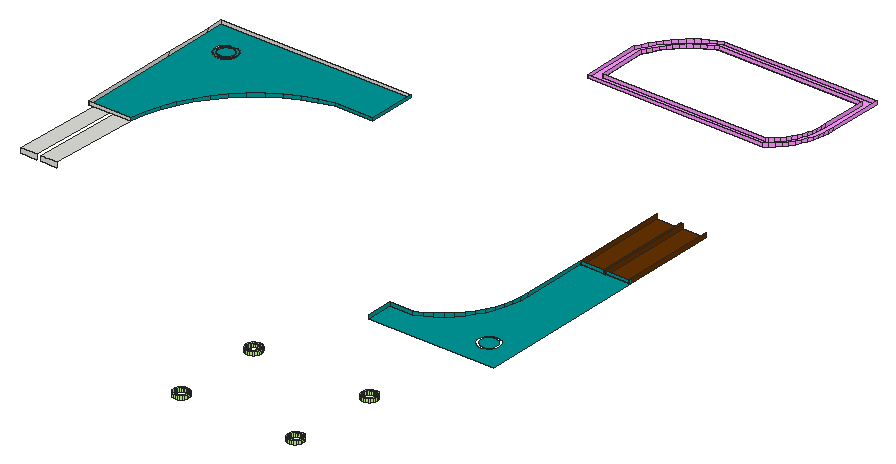
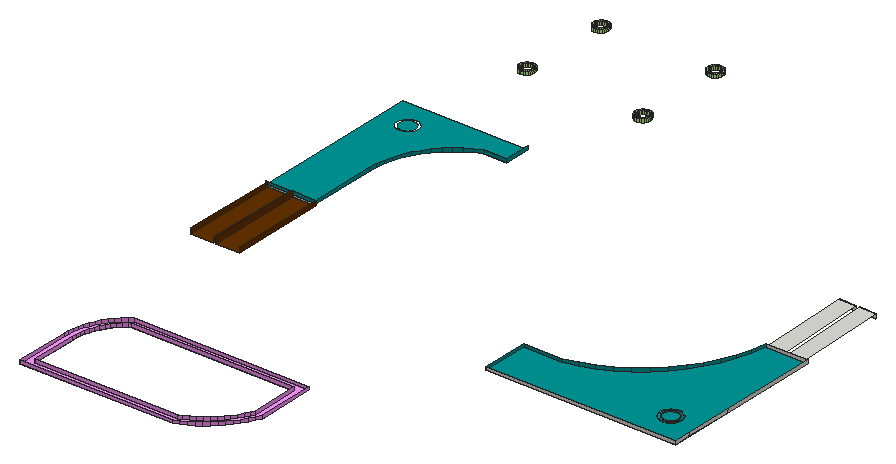
# SketchUp Ruby script. Lengths in inches.
U = 1.inch
M = Sketchup.active_model
def pt(a) = Geom::Point3d.new(a.map { |v| v * U })
def face(e, loops, mat)
  f = e.add_face(loops[0].map { |a| pt(a) })
  loops[1..].each { |l| e.add_face(l.map { |a| pt(a) }).erase! }
  f.material = f.back_material = mat if mat
  f
end
# faces: each face lists its corners as indices into pts; further lists are holes
def faces(e, pts, list, mat = nil) = list.each { |f| face(e, (f[0].is_a?(Array) ? f : [f]).map { |l| l.map { |i| pts[i] } }, mat) }
# xy, xz, yz: faces in a plane at the given z, y or x. An outline is a flat list of corners, or four numbers for a rectangle; further outlines are holes
def ring(l) = l.size == 4 ? [[l[0], l[1]], [l[2], l[1]], [l[2], l[3]], [l[0], l[3]]] : l.each_slice(2).to_a
def flat(e, list, mat, &to3) = list.each { |f| face(e, (f[0].is_a?(Array) ? f : [f]).map { |l| ring(l).map { |u, v| to3.(u, v) } }, mat) }
def xy(e, z, list, mat = nil) = flat(e, list, mat) { |x, y| [x, y, z] }
def xz(e, y, list, mat = nil) = flat(e, list, mat) { |x, z| [x, y, z] }
def yz(e, x, list, mat = nil) = flat(e, list, mat) { |y, z| [x, y, z] }
def lines(e, pts, list) = list.each { |a, b| e.add_line(pt(pts[a]), pt(pts[b])) }
# prism: a flat outline (further loops are holes) pulled along v
def prism(e, loops, v, mat = nil)
  f = face(e, loops, mat); d = Geom::Vector3d.new(v.map { |x| x * U })
  f.pushpull(f.normal.samedirection?(d) ? d.length : -d.length)
end
def box(e, o, s, mat = nil) = prism(e, [[o, [o[0] + s[0], o[1], o[2]], [o[0] + s[0], o[1] + s[1], o[2]], [o[0], o[1] + s[1], o[2]]]], [0, 0, s[2]], mat)
def at(x, y, z, deg = 0) = Geom::Transformation.translation(pt([x, y, z])) * Geom::Transformation.rotation(ORIGIN, Z_AXIS, deg.degrees)
def axes(o, x, y, z) = Geom::Transformation.new([*x, 0, *y, 0, *z, 0, *pt(o).to_a, 1])
def part(name) = M.definitions.add(name)
# library, detail: a bought-in or finely detailed component or shape, given as its bounding box
def library(name, o, s) = part(name).tap { |d| box(d.entities, o, s) }
def detail(e, o, s) = box(e.add_group.entities, o, s)
def put(e, d, t, mat = nil) = e.add_instance(d, t).tap { |i| i.material = mat if mat }
def group(e, t, mat = nil) = e.add_group.tap { |g| g.transformation = t; g.material = mat if mat }.entities
root = M.entities
M.materials.add("[Color C08]").color = [102, 51, 0]
M.materials.add("[Color F02]").color = [204, 255, 153]
M.materials.add("[Color H07]").color = [0, 153, 153]
M.materials.add("[Color K02]").color = [255, 153, 255]
M.materials.add("[Color M00]").color = [255, 255, 255]
M.materials.add("[Marble Carrara Gold Floor Tile]").color = [225, 223, 217]
xy(root,116.1875,[[418.74,309.14,433.17,368.58],[434.49,309.14,448.92,368.58]],"[Color C08]")
xy(root,116.1875,[[[153.48,358.9,151.72,358.91,150.02,359.37,148.49,360.26,147.25,361.51,146.375,363.04,145.93,364.74,145.93,366.51,146.4,368.21,147.28,369.73,148.53,370.97,150.0625,371.85,151.77,372.29,153.53,372.29,155.23,371.83,156.75,370.9375,157.99,369.6875,158.87,368.16,159.32,366.45,159.3125,364.69,158.85,362.99,157.96,361.47,156.71,360.23,155.18,359.35],[152.62,360.6,153.92,360.77,155.12,361.27,156.16,362.0625,156.95,363.1,157.45,364.31,157.62,365.6,157.45,366.89,156.95,368.1,156.16,369.13,155.12,369.93,153.92,370.43,152.62,370.6,151.33,370.43,150.12,369.93,149.09,369.13,148.29,368.1,147.79,366.89,147.62,365.6,147.79,364.31,148.29,363.1,149.09,362.0625,150.12,361.27,151.33,360.77]]],"[Color M00]")
xy(root,117.1875,[[[348.25,81.79,347.02,81.91,345.85,82.34,344.84,83.06,344.05,84.01,343.53,85.14,343.33,86.36,343.44,87.6,343.875,88.76,344.59,89.77,345.55,90.5625,346.68,91.08,347.9,91.29,349.13,91.17,350.29,90.74,351.31,90.02,352.1,89.07,352.61,87.9375,352.82,86.72,352.7,85.48,352.27,84.32,351.55,83.31,350.6,82.52,349.47,82],[348.07,83.14,348.95,83.26,349.77,83.6,350.48,84.14,351.02,84.84,351.36,85.66,351.47,86.54,351.36,87.42,351.02,88.24,350.48,88.94,349.77,89.48,348.95,89.82,348.07,89.9375,347.19,89.82,346.375,89.48,345.67,88.94,345.13,88.24,344.79,87.42,344.68,86.54,344.79,85.66,345.13,84.84,345.67,84.14,346.375,83.6,347.19,83.26]],[[419.3125,81.79,418.08,81.91,416.92,82.34,415.9,83.06,415.11,84.01,414.6,85.14,414.39,86.36,414.51,87.6,414.9375,88.76,415.66,89.77,416.61,90.5625,417.74,91.08,418.96,91.29,420.2,91.17,421.36,90.74,422.37,90.02,423.16,89.07,423.68,87.9375,423.88,86.72,423.77,85.48,423.33,84.32,422.62,83.31,421.66,82.52,420.53,82],[419.14,83.14,420.02,83.26,420.84,83.6,421.54,84.14,422.08,84.84,422.42,85.66,422.53,86.54,422.42,87.42,422.08,88.24,421.54,88.94,420.84,89.48,420.02,89.82,419.14,89.9375,418.26,89.82,417.4375,89.48,416.73,88.94,416.19,88.24,415.85,87.42,415.74,86.54,415.85,85.66,416.19,84.84,416.73,84.14,417.4375,83.6,418.26,83.26]],[[421.43,136.83,420.2,136.95,419.04,137.38,418.03,138.1,417.24,139.05,416.72,140.18,416.51,141.4,416.63,142.64,417.06,143.8,417.78,144.81,418.73,145.6,419.86,146.12,421.08,146.32,422.32,146.21,423.48,145.78,424.49,145.06,425.28,144.1,425.8,142.97,426.01,141.75,425.89,140.52,425.46,139.36,424.74,138.34,423.78,137.55,422.66,137.04],[421.26,138.18,422.14,138.29,422.96,138.63,423.66,139.17,424.2,139.88,424.54,140.7,424.66,141.58,424.54,142.46,424.2,143.28,423.66,143.98,422.96,144.52,422.14,144.86,421.26,144.97,420.38,144.86,419.56,144.52,418.86,143.98,418.32,143.28,417.98,142.46,417.86,141.58,417.98,140.7,418.32,139.88,418.86,139.17,419.56,138.63,420.38,138.29]],[[348.25,138.17,347.02,138.28,345.85,138.72,344.84,139.43,344.05,140.39,343.53,141.52,343.33,142.74,343.44,143.97,343.875,145.14,344.59,146.15,345.55,146.9375,346.68,147.45,347.9,147.66,349.13,147.55,350.29,147.11,351.31,146.4,352.1,145.44,352.61,144.3125,352.82,143.09,352.7,141.86,352.27,140.69,351.55,139.68,350.6,138.89,349.47,138.375],[348.07,139.52,348.95,139.63,349.77,139.97,350.48,140.51,351.02,141.22,351.36,142.04,351.47,142.91,351.36,143.79,351.02,144.61,350.48,145.32,349.77,145.86,348.95,146.2,348.07,146.3125,347.19,146.2,346.375,145.86,345.67,145.32,345.13,144.61,344.79,143.79,344.68,142.91,344.79,142.04,345.13,141.22,345.67,140.51,346.375,139.97,347.19,139.63]]],"[Color F02]")
xy(root,117.1875,[[[371.8,202.59,371.8,218.96,386.375,218.96,391.03,221.23,395.45,223.95,399.59,227.09,403.4,230.61,406.85,234.48,409.91,238.67,412.55,243.13,414.74,247.83,416.47,252.72,417.72,257.76,418.47,262.89,418.72,268.07,418.72,309.14,449.85,309.14,449.85,202.59],[433.35,213.79,435.05,214.24,436.58,215.12,437.83,216.36,438.72,217.88,439.18,219.58,439.19,221.35,438.74,223.05,437.87,224.58,436.625,225.83,435.1,226.72,433.4,227.18,431.64,227.19,429.94,226.74,428.41,225.86,427.16,224.62,426.27,223.1,425.81,221.4,425.8,219.63,426.25,217.93,427.125,216.4,428.36,215.15,429.89,214.26,431.59,213.8]],[432.49,215.49,431.2,215.66,429.99,216.16,428.96,216.95,428.16,217.99,427.66,219.2,427.49,220.49,427.66,221.78,428.16,222.99,428.96,224.03,429.99,224.82,431.2,225.32,432.49,225.49,433.79,225.32,434.99,224.82,436.03,224.03,436.82,222.99,437.32,221.78,437.49,220.49,437.32,219.2,436.82,217.99,436.03,216.95,434.99,216.16,433.79,215.66],[[133.15,283.41,133.15,386.28,251.25,386.28,251.25,356.85,227.25,356.85,218.64,354.61,210.31,351.49,202.34,347.53,194.83,342.76,187.85,337.25,181.48,331.04,175.78,324.21,170.82,316.82,166.65,308.96,163.32,300.72,160.85,292.17,159.28,283.41],[153.48,358.9,155.18,359.35,156.71,360.23,157.96,361.47,158.85,362.99,159.3125,364.69,159.32,366.45,158.87,368.16,157.99,369.6875,156.75,370.9375,155.23,371.83,153.53,372.29,151.77,372.29,150.0625,371.85,148.53,370.97,147.28,369.73,146.4,368.21,145.93,366.51,145.93,364.74,146.375,363.04,147.25,361.51,148.49,360.26,150.02,359.37,151.72,358.91]],[[153.48,358.9,155.18,359.35,156.71,360.23,157.96,361.47,158.85,362.99,159.3125,364.69,159.32,366.45,158.87,368.16,157.99,369.6875,156.75,370.9375,155.23,371.83,153.53,372.29,151.77,372.29,150.0625,371.85,148.53,370.97,147.28,369.73,146.4,368.21,145.93,366.51,145.93,364.74,146.375,363.04,147.25,361.51,148.49,360.26,150.02,359.37,151.72,358.91],[152.62,360.6,151.33,360.77,150.12,361.27,149.09,362.0625,148.29,363.1,147.79,364.31,147.62,365.6,147.79,366.89,148.29,368.1,149.09,369.13,150.12,369.93,151.33,370.43,152.62,370.6,153.92,370.43,155.12,369.93,156.16,369.13,156.95,368.1,157.45,366.89,157.62,365.6,157.45,364.31,156.95,363.1,156.16,362.0625,155.12,361.27,153.92,360.77]],[152.62,360.6,151.33,360.77,150.12,361.27,149.09,362.0625,148.29,363.1,147.79,364.31,147.62,365.6,147.79,366.89,148.29,368.1,149.09,369.13,150.12,369.93,151.33,370.43,152.62,370.6,153.92,370.43,155.12,369.93,156.16,369.13,156.95,368.1,157.45,366.89,157.62,365.6,157.45,364.31,156.95,363.1,156.16,362.0625,155.12,361.27,153.92,360.77]],"[Color H07]")
xy(root,117.1875,[[[306.15,455.42,306.15,491.45,307.65,494.89,309.39,498.21,311.35,501.41,313.52,504.47,315.89,507.38,318.45,510.12,321.1875,512.68,324.1,515.05,327.16,517.22,330.36,519.18,333.68,520.92,337.12,522.42,432.08,522.42,432.08,488.92,431.95,485.67,431.57,482.43,430.93,479.23,430.04,476.1,428.9,473.04,427.52,470.09,425.92,467.25,424.1,464.55,422.07,462,419.84,459.62,417.43,457.42,414.86,455.42],[311.23,460.51,413.12,460.51,414.15,461.3125,416.27,463.24,418.22,465.33,420,467.5625,421.59,469.93,423,472.42,424.2,475.01,425.2,477.68,425.98,480.43,426.54,483.23,426.88,486.07,427,489.02,427,517.34,338.18,517.34,335.88,516.33,332.86,514.75,329.96,512.97,327.18,511,324.53,508.85,322.05,506.52,319.72,504.03,317.57,501.39,315.59,498.61,313.82,495.71,312.24,492.6875,311.23,490.39]]],"[Color K02]")
xz(root,218.96,[[371.8,117.1875,386.375,119.1875]],"[Color H07]")
xz(root,283.41,[[133.15,117.1875,159.28,119.1875]],"[Marble Carrara Gold Floor Tile]")
xz(root,309.14,[[418.72,117.1875,418.74,119.1875],[418.74,117.1875,433.17,119.1875],[433.17,117.1875,434.49,119.1875],[434.49,117.1875,448.92,119.1875],[448.92,117.1875,449.85,119.1875]],"[Color H07]")
xz(root,309.14,[[418.74,116.1875,433.17,117.1875],[434.49,116.1875,448.92,117.1875]],"[Marble Carrara Gold Floor Tile]")
xz(root,356.85,[[227.25,117.1875,251.25,119.1875]],"[Color H07]")
xz(root,372.29,[[151.77,116.1875,153.53,117.1875]],"[Color M00]")
xz(root,386.28,[[133.15,117.1875,251.25,119.1875]],"[Marble Carrara Gold Floor Tile]")
xz(root,455.42,[[306.15,117.1875,414.86,119.1875]],"[Color K02]")
xz(root,460.51,[[311.23,117.1875,413.12,119.1875]],"[Color K02]")
xz(root,517.34,[[338.18,117.1875,427,119.1875]],"[Color K02]")
xz(root,522.42,[[337.12,117.1875,432.08,119.1875]],"[Color K02]")
yz(root,133.15,[[283.41,117.1875,345.53,119.1875],[345.53,117.1875,375.53,119.1875],[375.53,117.1875,386.28,119.1875]],"[Marble Carrara Gold Floor Tile]")
yz(root,145.93,[[364.74,116.1875,366.51,117.1875]],"[Color M00]")
yz(root,251.25,[[356.85,117.1875,386.28,119.1875]],"[Color H07]")
yz(root,306.15,[[455.42,117.1875,491.45,119.1875]],"[Color K02]")
yz(root,311.23,[[460.51,117.1875,490.39,119.1875]],"[Color K02]")
yz(root,371.8,[[202.59,117.1875,218.96,119.1875]],"[Color H07]")
yz(root,418.72,[[268.07,117.1875,309.14,119.1875]],"[Color H07]")
yz(root,418.74,[[309.14,116.1875,368.58,119.1875]],"[Color C08]")
yz(root,427,[[489.02,117.1875,517.34,119.1875]],"[Color K02]")
yz(root,432.08,[[488.92,117.1875,522.42,119.1875]],"[Color K02]")
yz(root,433.17,[[309.14,116.1875,368.58,119.1875]],"[Color C08]")
yz(root,434.49,[[309.14,116.1875,368.58,119.1875]],"[Color C08]")
yz(root,448.92,[[309.14,116.1875,368.58,119.1875]],"[Color C08]")
p = [[146.22,226.59,119.1875],[135.92,226.59,119.1875],[135.92,226.48,116.1875],[146.22,226.48,116.1875],[158.84,226.59,119.1875],[148.55,226.59,119.1875],
  [148.55,226.48,116.1875],[158.84,226.48,116.1875],[151.72,358.91,117.1875],[150.02,359.37,117.1875],[150.02,359.37,116.1875],[151.72,358.91,116.1875],
  [153.48,358.9,117.1875],[153.48,358.9,116.1875],[155.18,359.35,117.1875],[155.18,359.35,116.1875],[148.49,360.26,117.1875],[148.49,360.26,116.1875],
  [156.71,360.23,117.1875],[156.71,360.23,116.1875],[157.96,361.47,117.1875],[157.96,361.47,116.1875],[147.25,361.51,117.1875],[147.25,361.51,116.1875],
  [151.33,360.77,117.1875],[152.62,360.6,117.1875],[152.62,360.6,116.1875],[151.33,360.77,116.1875],[153.92,360.77,117.1875],[153.92,360.77,116.1875],
  [150.12,361.27,117.1875],[150.12,361.27,116.1875],[155.12,361.27,117.1875],[155.12,361.27,116.1875],[149.09,362.0625,117.1875],[149.09,362.0625,116.1875],
  [156.16,362.0625,117.1875],[156.16,362.0625,116.1875],[146.375,363.04,117.1875],[146.375,363.04,116.1875],[158.85,362.99,117.1875],[158.85,362.99,116.1875],
  [148.29,363.1,117.1875],[148.29,363.1,116.1875],[156.95,363.1,117.1875],[156.95,363.1,116.1875],[145.93,364.74,117.1875],[145.93,364.74,116.1875],
  [159.3125,364.69,117.1875],[159.3125,364.69,116.1875],[147.79,364.31,117.1875],[147.79,364.31,116.1875],[157.45,364.31,117.1875],[157.45,364.31,116.1875],
  [147.62,365.6,117.1875],[147.62,365.6,116.1875],[157.62,365.6,117.1875],[157.62,365.6,116.1875],[159.32,366.45,117.1875],[159.32,366.45,116.1875],
  [147.79,366.89,117.1875],[147.79,366.89,116.1875],[157.45,366.89,117.1875],[157.45,366.89,116.1875],[145.93,366.51,117.1875],[146.4,368.21,117.1875],
  [146.4,368.21,116.1875],[145.93,366.51,116.1875],[158.87,368.16,117.1875],[158.87,368.16,116.1875],[148.29,368.1,117.1875],[148.29,368.1,116.1875],
  [156.95,368.1,117.1875],[156.95,368.1,116.1875],[149.09,369.13,117.1875],[149.09,369.13,116.1875],[156.16,369.13,117.1875],[156.16,369.13,116.1875],
  [147.28,369.73,117.1875],[147.28,369.73,116.1875],[157.99,369.6875,117.1875],[157.99,369.6875,116.1875],[150.12,369.93,117.1875],[150.12,369.93,116.1875],
  [155.12,369.93,117.1875],[155.12,369.93,116.1875],[148.53,370.97,117.1875],[148.53,370.97,116.1875],[156.75,370.9375,117.1875],[156.75,370.9375,116.1875],
  [151.33,370.43,117.1875],[151.33,370.43,116.1875],[153.92,370.43,117.1875],[153.92,370.43,116.1875],[152.62,370.6,117.1875],[152.62,370.6,116.1875],
  [155.23,371.83,117.1875],[155.23,371.83,116.1875],[150.0625,371.85,117.1875],[150.0625,371.85,116.1875],[151.77,372.29,117.1875],[151.77,372.29,116.1875],
  [153.53,372.29,117.1875],[153.53,372.29,116.1875],[135.92,287.31,116.99],[146.22,287.31,116.99],[148.55,286.68,117.02],[158.84,286.68,117.02],
  [348.25,81.79,119.1875],[347.02,81.91,119.1875],[347.02,81.91,117.1875],[348.25,81.79,117.1875],[349.47,82,119.1875],[349.47,82,117.1875],
  [419.3125,81.79,119.1875],[418.08,81.91,119.1875],[418.08,81.91,117.1875],[419.3125,81.79,117.1875],[420.53,82,119.1875],[420.53,82,117.1875],
  [345.85,82.34,119.1875],[345.85,82.34,117.1875],[416.92,82.34,119.1875],[416.92,82.34,117.1875],[350.6,82.52,119.1875],[350.6,82.52,117.1875],
  [421.66,82.52,119.1875],[421.66,82.52,117.1875],[344.84,83.06,119.1875],[344.84,83.06,117.1875],[415.9,83.06,119.1875],[415.9,83.06,117.1875],
  [351.55,83.31,119.1875],[351.55,83.31,117.1875],[422.62,83.31,119.1875],[422.62,83.31,117.1875],[344.05,84.01,119.1875],[344.05,84.01,117.1875],
  [347.19,83.26,119.1875],[348.07,83.14,119.1875],[348.07,83.14,117.1875],[347.19,83.26,117.1875],[348.95,83.26,119.1875],[348.95,83.26,117.1875],
  [415.11,84.01,119.1875],[415.11,84.01,117.1875],[418.26,83.26,119.1875],[419.14,83.14,119.1875],[419.14,83.14,117.1875],[418.26,83.26,117.1875],
  [420.02,83.26,119.1875],[420.02,83.26,117.1875],[346.375,83.6,119.1875],[346.375,83.6,117.1875],[349.77,83.6,119.1875],[349.77,83.6,117.1875],
  [352.27,84.32,119.1875],[352.27,84.32,117.1875],[417.4375,83.6,119.1875],[417.4375,83.6,117.1875],[420.84,83.6,119.1875],[420.84,83.6,117.1875],
  [423.33,84.32,119.1875],[423.33,84.32,117.1875],[345.67,84.14,119.1875],[345.67,84.14,117.1875],[350.48,84.14,119.1875],[350.48,84.14,117.1875],
  [416.73,84.14,119.1875],[416.73,84.14,117.1875],[421.54,84.14,119.1875],[421.54,84.14,117.1875],[343.53,85.14,119.1875],[343.53,85.14,117.1875],
  [414.6,85.14,119.1875],[414.6,85.14,117.1875],[345.13,84.84,119.1875],[345.13,84.84,117.1875],[351.02,84.84,119.1875],[351.02,84.84,117.1875],
  [416.19,84.84,119.1875],[416.19,84.84,117.1875],[422.08,84.84,119.1875],[422.08,84.84,117.1875],[352.7,85.48,119.1875],[352.7,85.48,117.1875],
  [423.77,85.48,119.1875],[423.77,85.48,117.1875],[344.79,85.66,119.1875],[344.79,85.66,117.1875],[351.36,85.66,119.1875],[351.36,85.66,117.1875],
  [415.85,85.66,119.1875],[415.85,85.66,117.1875],[422.42,85.66,119.1875],[422.42,85.66,117.1875],[343.33,86.36,119.1875],[343.33,86.36,117.1875],
  [414.39,86.36,119.1875],[414.39,86.36,117.1875],[352.82,86.72,119.1875],[352.82,86.72,117.1875],[423.88,86.72,119.1875],[423.88,86.72,117.1875],
  [344.68,86.54,119.1875],[344.68,86.54,117.1875],[351.47,86.54,119.1875],[351.47,86.54,117.1875],[415.74,86.54,119.1875],[415.74,86.54,117.1875],
  [422.53,86.54,119.1875],[422.53,86.54,117.1875],[343.44,87.6,119.1875],[343.44,87.6,117.1875],[414.51,87.6,119.1875],[414.51,87.6,117.1875],
  [344.79,87.42,119.1875],[344.79,87.42,117.1875],[351.36,87.42,119.1875],[351.36,87.42,117.1875],[415.85,87.42,119.1875],[415.85,87.42,117.1875],
  [422.42,87.42,119.1875],[422.42,87.42,117.1875],[352.61,87.9375,119.1875],[352.61,87.9375,117.1875],[423.68,87.9375,119.1875],[423.68,87.9375,117.1875],
  [345.13,88.24,119.1875],[345.13,88.24,117.1875],[351.02,88.24,119.1875],[351.02,88.24,117.1875],[416.19,88.24,119.1875],[416.19,88.24,117.1875],
  [422.08,88.24,119.1875],[422.08,88.24,117.1875],[343.875,88.76,119.1875],[343.875,88.76,117.1875],[414.9375,88.76,119.1875],[414.9375,88.76,117.1875],
  [352.1,89.07,119.1875],[352.1,89.07,117.1875],[423.16,89.07,119.1875],[423.16,89.07,117.1875],[345.67,88.94,119.1875],[345.67,88.94,117.1875],
  [350.48,88.94,119.1875],[350.48,88.94,117.1875],[416.73,88.94,119.1875],[416.73,88.94,117.1875],[421.54,88.94,119.1875],[421.54,88.94,117.1875],
  [344.59,89.77,119.1875],[344.59,89.77,117.1875],[415.66,89.77,119.1875],[415.66,89.77,117.1875],[346.375,89.48,119.1875],[346.375,89.48,117.1875],
  [349.77,89.48,119.1875],[349.77,89.48,117.1875],[417.4375,89.48,119.1875],[417.4375,89.48,117.1875],[420.84,89.48,119.1875],[420.84,89.48,117.1875],
  [351.31,90.02,119.1875],[351.31,90.02,117.1875],[422.37,90.02,119.1875],[422.37,90.02,117.1875],[347.19,89.82,119.1875],[347.19,89.82,117.1875],
  [348.95,89.82,119.1875],[348.95,89.82,117.1875],[418.26,89.82,119.1875],[418.26,89.82,117.1875],[420.02,89.82,119.1875],[420.02,89.82,117.1875],
  [345.55,90.5625,119.1875],[345.55,90.5625,117.1875],[348.07,89.9375,119.1875],[348.07,89.9375,117.1875],[416.61,90.5625,119.1875],[416.61,90.5625,117.1875],
  [419.14,89.9375,119.1875],[419.14,89.9375,117.1875],[350.29,90.74,119.1875],[350.29,90.74,117.1875],[421.36,90.74,119.1875],[421.36,90.74,117.1875],
  [346.68,91.08,119.1875],[346.68,91.08,117.1875],[417.74,91.08,119.1875],[417.74,91.08,117.1875],[349.13,91.17,119.1875],[349.13,91.17,117.1875],
  [420.2,91.17,119.1875],[420.2,91.17,117.1875],[347.9,91.29,119.1875],[347.9,91.29,117.1875],[418.96,91.29,119.1875],[418.96,91.29,117.1875],
  [421.43,136.83,119.1875],[420.2,136.95,119.1875],[420.2,136.95,117.1875],[421.43,136.83,117.1875],[422.66,137.04,119.1875],[422.66,137.04,117.1875],
  [419.04,137.38,119.1875],[419.04,137.38,117.1875],[423.78,137.55,119.1875],[423.78,137.55,117.1875],[418.03,138.1,119.1875],[418.03,138.1,117.1875],
  [424.74,138.34,119.1875],[424.74,138.34,117.1875],[417.24,139.05,119.1875],[417.24,139.05,117.1875],[348.25,138.17,119.1875],[347.02,138.28,119.1875],
  [347.02,138.28,117.1875],[348.25,138.17,117.1875],[349.47,138.375,119.1875],[349.47,138.375,117.1875],[420.38,138.29,119.1875],[421.26,138.18,119.1875],
  [421.26,138.18,117.1875],[420.38,138.29,117.1875],[422.14,138.29,119.1875],[422.14,138.29,117.1875],[345.85,138.72,119.1875],[345.85,138.72,117.1875],
  [419.56,138.63,119.1875],[419.56,138.63,117.1875],[422.96,138.63,119.1875],[422.96,138.63,117.1875],[425.46,139.36,119.1875],[425.46,139.36,117.1875],
  [350.6,138.89,119.1875],[350.6,138.89,117.1875],[418.86,139.17,119.1875],[418.86,139.17,117.1875],[423.66,139.17,119.1875],[423.66,139.17,117.1875],
  [344.84,139.43,119.1875],[344.84,139.43,117.1875],[351.55,139.68,119.1875],[351.55,139.68,117.1875],[416.72,140.18,119.1875],[416.72,140.18,117.1875],
  [418.32,139.88,119.1875],[418.32,139.88,117.1875],[424.2,139.88,119.1875],[424.2,139.88,117.1875],[344.05,140.39,119.1875],[344.05,140.39,117.1875],
  [425.89,140.52,119.1875],[425.89,140.52,117.1875],[347.19,139.63,119.1875],[348.07,139.52,119.1875],[348.07,139.52,117.1875],[347.19,139.63,117.1875],
  [348.95,139.63,119.1875],[348.95,139.63,117.1875],[346.375,139.97,119.1875],[346.375,139.97,117.1875],[349.77,139.97,119.1875],[349.77,139.97,117.1875],
  [352.27,140.69,119.1875],[352.27,140.69,117.1875],[417.98,140.7,119.1875],[417.98,140.7,117.1875],[424.54,140.7,119.1875],[424.54,140.7,117.1875],
  [345.67,140.51,119.1875],[345.67,140.51,117.1875],[350.48,140.51,119.1875],[350.48,140.51,117.1875],[416.51,141.4,119.1875],[416.51,141.4,117.1875],
  [343.53,141.52,119.1875],[343.53,141.52,117.1875],[345.13,141.22,119.1875],[345.13,141.22,117.1875],[351.02,141.22,119.1875],[351.02,141.22,117.1875],
  [426.01,141.75,119.1875],[426.01,141.75,117.1875],[352.7,141.86,119.1875],[352.7,141.86,117.1875],[417.86,141.58,119.1875],[417.86,141.58,117.1875],
  [424.66,141.58,119.1875],[424.66,141.58,117.1875],[344.79,142.04,119.1875],[344.79,142.04,117.1875],[351.36,142.04,119.1875],[351.36,142.04,117.1875],
  [416.63,142.64,119.1875],[416.63,142.64,117.1875],[343.33,142.74,119.1875],[343.33,142.74,117.1875],[417.98,142.46,119.1875],[417.98,142.46,117.1875],
  [424.54,142.46,119.1875],[424.54,142.46,117.1875],[425.8,142.97,119.1875],[425.8,142.97,117.1875],[352.82,143.09,119.1875],[352.82,143.09,117.1875],
  [344.68,142.91,119.1875],[344.68,142.91,117.1875],[351.47,142.91,119.1875],[351.47,142.91,117.1875],[418.32,143.28,119.1875],[418.32,143.28,117.1875],
  [424.2,143.28,119.1875],[424.2,143.28,117.1875],[417.06,143.8,119.1875],[417.06,143.8,117.1875],[343.44,143.97,119.1875],[343.44,143.97,117.1875],
  [344.79,143.79,119.1875],[344.79,143.79,117.1875],[351.36,143.79,119.1875],[351.36,143.79,117.1875],[425.28,144.1,119.1875],[425.28,144.1,117.1875],
  [352.61,144.3125,119.1875],[352.61,144.3125,117.1875],[418.86,143.98,119.1875],[418.86,143.98,117.1875],[423.66,143.98,119.1875],[423.66,143.98,117.1875],
  [345.13,144.61,119.1875],[345.13,144.61,117.1875],[351.02,144.61,119.1875],[351.02,144.61,117.1875],[417.78,144.81,119.1875],[417.78,144.81,117.1875],
  [343.875,145.14,119.1875],[343.875,145.14,117.1875],[419.56,144.52,119.1875],[419.56,144.52,117.1875],[422.96,144.52,119.1875],[422.96,144.52,117.1875],
  [424.49,145.06,119.1875],[424.49,145.06,117.1875],[352.1,145.44,119.1875],[352.1,145.44,117.1875],[420.38,144.86,119.1875],[420.38,144.86,117.1875],
  [422.14,144.86,119.1875],[422.14,144.86,117.1875],[345.67,145.32,119.1875],[345.67,145.32,117.1875],[350.48,145.32,119.1875],[350.48,145.32,117.1875],
  [418.73,145.6,119.1875],[418.73,145.6,117.1875],[421.26,144.97,119.1875],[421.26,144.97,117.1875],[344.59,146.15,119.1875],[344.59,146.15,117.1875],
  [423.48,145.78,119.1875],[423.48,145.78,117.1875],[346.375,145.86,119.1875],[346.375,145.86,117.1875],[349.77,145.86,119.1875],[349.77,145.86,117.1875],
  [351.31,146.4,119.1875],[351.31,146.4,117.1875],[419.86,146.12,119.1875],[419.86,146.12,117.1875],[422.32,146.21,119.1875],[422.32,146.21,117.1875],
  [347.19,146.2,119.1875],[347.19,146.2,117.1875],[348.95,146.2,119.1875],[348.95,146.2,117.1875],[345.55,146.9375,119.1875],[345.55,146.9375,117.1875],
  [421.08,146.32,119.1875],[421.08,146.32,117.1875],[348.07,146.3125,119.1875],[348.07,146.3125,117.1875],[350.29,147.11,119.1875],[350.29,147.11,117.1875],
  [346.68,147.45,119.1875],[346.68,147.45,117.1875],[349.13,147.55,119.1875],[349.13,147.55,117.1875],[347.9,147.66,119.1875],[347.9,147.66,117.1875],
  [386.375,218.96,119.1875],[391.03,221.23,119.1875],[391.03,221.23,117.1875],[386.375,218.96,117.1875],[395.45,223.95,119.1875],[395.45,223.95,117.1875],
  [399.59,227.09,119.1875],[399.59,227.09,117.1875],[403.4,230.61,119.1875],[403.4,230.61,117.1875],[406.85,234.48,119.1875],[406.85,234.48,117.1875],
  [409.91,238.67,119.1875],[409.91,238.67,117.1875],[412.55,243.13,119.1875],[412.55,243.13,117.1875],[414.74,247.83,119.1875],[414.74,247.83,117.1875],
  [416.47,252.72,119.1875],[416.47,252.72,117.1875],[417.72,257.76,119.1875],[417.72,257.76,117.1875],[418.47,262.89,119.1875],[418.47,262.89,117.1875],
  [418.72,268.07,119.1875],[418.72,268.07,117.1875],[160.85,292.17,119.1875],[159.28,283.41,119.1875],[159.28,283.41,117.1875],[160.85,292.17,117.1875],
  [163.32,300.72,119.1875],[163.32,300.72,117.1875],[166.65,308.96,119.1875],[166.65,308.96,117.1875],[170.82,316.82,119.1875],[170.82,316.82,117.1875],
  [175.78,324.21,119.1875],[175.78,324.21,117.1875],[181.48,331.04,119.1875],[181.48,331.04,117.1875],[187.85,337.25,119.1875],[187.85,337.25,117.1875],
  [194.83,342.76,119.1875],[194.83,342.76,117.1875],[202.34,347.53,119.1875],[202.34,347.53,117.1875],[210.31,351.49,119.1875],[210.31,351.49,117.1875],
  [218.64,354.61,119.1875],[218.64,354.61,117.1875],[227.25,356.85,119.1875],[227.25,356.85,117.1875],[417.43,457.42,119.1875],[414.86,455.42,119.1875],
  [414.86,455.42,117.1875],[417.43,457.42,117.1875],[419.84,459.62,119.1875],[419.84,459.62,117.1875],[422.07,462,119.1875],[422.07,462,117.1875],
  [413.12,460.51,119.1875],[414.15,461.3125,119.1875],[414.15,461.3125,117.1875],[413.12,460.51,117.1875],[416.27,463.24,119.1875],[416.27,463.24,117.1875],
  [424.1,464.55,119.1875],[424.1,464.55,117.1875],[418.22,465.33,119.1875],[418.22,465.33,117.1875],[425.92,467.25,119.1875],[425.92,467.25,117.1875],
  [420,467.5625,119.1875],[420,467.5625,117.1875],[427.52,470.09,119.1875],[427.52,470.09,117.1875],[421.59,469.93,119.1875],[421.59,469.93,117.1875],
  [423,472.42,119.1875],[423,472.42,117.1875],[428.9,473.04,119.1875],[428.9,473.04,117.1875],[424.2,475.01,119.1875],[424.2,475.01,117.1875],
  [430.04,476.1,119.1875],[430.04,476.1,117.1875],[425.2,477.68,119.1875],[425.2,477.68,117.1875],[430.93,479.23,119.1875],[430.93,479.23,117.1875],
  [425.98,480.43,119.1875],[425.98,480.43,117.1875],[431.57,482.43,119.1875],[431.57,482.43,117.1875],[426.54,483.23,119.1875],[426.54,483.23,117.1875],
  [431.95,485.67,119.1875],[431.95,485.67,117.1875],[426.88,486.07,119.1875],[426.88,486.07,117.1875],[432.08,488.92,119.1875],[432.08,488.92,117.1875],
  [427,489.02,119.1875],[427,489.02,117.1875],[312.24,492.6875,119.1875],[311.23,490.39,119.1875],[311.23,490.39,117.1875],[312.24,492.6875,117.1875],
  [306.15,491.45,119.1875],[307.65,494.89,119.1875],[307.65,494.89,117.1875],[306.15,491.45,117.1875],[313.82,495.71,119.1875],[313.82,495.71,117.1875],
  [309.39,498.21,119.1875],[309.39,498.21,117.1875],[315.59,498.61,119.1875],[315.59,498.61,117.1875],[311.35,501.41,119.1875],[311.35,501.41,117.1875],
  [317.57,501.39,119.1875],[317.57,501.39,117.1875],[313.52,504.47,119.1875],[313.52,504.47,117.1875],[319.72,504.03,119.1875],[319.72,504.03,117.1875],
  [322.05,506.52,119.1875],[322.05,506.52,117.1875],[315.89,507.38,119.1875],[315.89,507.38,117.1875],[324.53,508.85,119.1875],[324.53,508.85,117.1875],
  [318.45,510.12,119.1875],[318.45,510.12,117.1875],[327.18,511,119.1875],[327.18,511,117.1875],[321.1875,512.68,119.1875],[321.1875,512.68,117.1875],
  [329.96,512.97,119.1875],[329.96,512.97,117.1875],[324.1,515.05,119.1875],[324.1,515.05,117.1875],[332.86,514.75,119.1875],[332.86,514.75,117.1875],
  [335.88,516.33,119.1875],[335.88,516.33,117.1875],[327.16,517.22,119.1875],[327.16,517.22,117.1875],[338.18,517.34,119.1875],[338.18,517.34,117.1875],
  [330.36,519.18,119.1875],[330.36,519.18,117.1875],[333.68,520.92,119.1875],[333.68,520.92,117.1875],[337.12,522.42,119.1875],[337.12,522.42,117.1875]]
faces(root,p,[[0,1,2,3],[4,5,6,7],[104,1,0,105],[106,5,4,107]])
faces(root,p,[[8,9,10,11],[12,8,11,13],[14,12,13,15],[9,16,17,10],[18,14,15,19],[20,18,19,21],[16,22,23,17],[22,38,39,23],
  [40,20,21,41],[38,46,47,39],[48,40,41,49],[58,48,49,59],[64,65,66,67],[68,58,59,69],[65,78,79,66],[80,68,69,81],
  [78,86,87,79],[88,80,81,89],[96,88,89,97],[86,98,99,87],[98,100,101,99],[102,96,97,103]],"[Color M00]")
faces(root,p,[[24,25,26,27],[25,28,29,26],[30,24,27,31],[28,32,33,29],[34,30,31,35],[32,36,37,33],[42,34,35,43],[36,44,45,37],
  [50,42,43,51],[44,52,53,45],[54,50,51,55],[52,56,57,53],[60,54,55,61],[56,62,63,57],[70,60,61,71],[62,72,73,63],
  [74,70,71,75],[72,76,77,73],[82,74,75,83],[76,84,85,77],[90,82,83,91],[84,92,93,85],[94,90,91,95],[92,94,95,93],
  [492,493,494,495],[493,496,497,494],[496,498,499,497],[498,500,501,499],[500,502,503,501],[502,504,505,503],[504,506,507,505],[506,508,509,507],
  [508,510,511,509],[510,512,513,511],[512,514,515,513],[514,516,517,515],[518,519,520,521],[522,518,521,523],[524,522,523,525],[526,524,525,527],
  [528,526,527,529],[530,528,529,531],[532,530,531,533],[534,532,533,535],[536,534,535,537],[538,536,537,539],[540,538,539,541],[542,540,541,543]],"[Color H07]")
faces(root,p,[[108,109,110,111],[112,108,111,113],[114,115,116,117],[118,114,117,119],[109,120,121,110],[115,122,123,116],[124,112,113,125],[126,118,119,127],
  [120,128,129,121],[122,130,131,123],[132,124,125,133],[134,126,127,135],[128,136,137,129],[138,139,140,141],[139,142,143,140],[130,144,145,131],
  [146,147,148,149],[147,150,151,148],[152,138,141,153],[142,154,155,143],[156,132,133,157],[158,146,149,159],[150,160,161,151],[162,134,135,163],
  [164,152,153,165],[154,166,167,155],[168,158,159,169],[160,170,171,161],[136,172,173,137],[144,174,175,145],[176,164,165,177],[166,178,179,167],
  [180,168,169,181],[170,182,183,171],[184,156,157,185],[186,162,163,187],[188,176,177,189],[178,190,191,179],[192,180,181,193],[182,194,195,183],
  [172,196,197,173],[174,198,199,175],[200,184,185,201],[202,186,187,203],[204,188,189,205],[190,206,207,191],[208,192,193,209],[194,210,211,195],
  [196,212,213,197],[198,214,215,199],[216,204,205,217],[206,218,219,207],[220,208,209,221],[210,222,223,211],[224,200,201,225],[226,202,203,227],
  [228,216,217,229],[218,230,231,219],[232,220,221,233],[222,234,235,223],[212,236,237,213],[214,238,239,215],[240,224,225,241],[242,226,227,243],
  [244,228,229,245],[230,246,247,231],[248,232,233,249],[234,250,251,235],[236,252,253,237],[238,254,255,239],[256,244,245,257],[246,258,259,247],
  [260,248,249,261],[250,262,263,251],[264,240,241,265],[266,242,243,267],[268,256,257,269],[258,270,271,259],[272,260,261,273],[262,274,275,263],
  [252,276,277,253],[278,268,269,279],[270,278,279,271],[254,280,281,255],[282,272,273,283],[274,282,283,275],[284,264,265,285],[286,266,267,287],
  [276,288,289,277],[280,290,291,281],[292,284,285,293],[294,286,287,295],[288,296,297,289],[290,298,299,291],[296,292,293,297],[298,294,295,299],
  [300,301,302,303],[304,300,303,305],[301,306,307,302],[308,304,305,309],[306,310,311,307],[312,308,309,313],[310,314,315,311],[316,317,318,319],
  [320,316,319,321],[322,323,324,325],[323,326,327,324],[317,328,329,318],[330,322,325,331],[326,332,333,327],[334,312,313,335],[336,320,321,337],
  [338,330,331,339],[332,340,341,333],[328,342,343,329],[344,336,337,345],[314,346,347,315],[348,338,339,349],[340,350,351,341],[342,352,353,343],
  [354,334,335,355],[356,357,358,359],[357,360,361,358],[362,356,359,363],[360,364,365,361],[366,344,345,367],[368,348,349,369],[350,370,371,351],
  [372,362,363,373],[364,374,375,365],[346,376,377,347],[352,378,379,353],[380,372,373,381],[374,382,383,375],[384,354,355,385],[386,366,367,387],
  [388,368,369,389],[370,390,391,371],[392,380,381,393],[382,394,395,383],[376,396,397,377],[378,398,399,379],[400,388,389,401],[390,402,403,391],
  [404,384,385,405],[406,386,387,407],[408,392,393,409],[394,410,411,395],[412,400,401,413],[402,414,415,403],[396,416,417,397],[398,418,419,399],
  [420,408,409,421],[410,422,423,411],[424,404,405,425],[426,406,407,427],[428,412,413,429],[414,430,431,415],[432,420,421,433],[422,434,435,423],
  [416,436,437,417],[418,438,439,419],[440,428,429,441],[430,442,443,431],[444,424,425,445],[446,426,427,447],[448,440,441,449],[442,450,451,443],
  [452,432,433,453],[434,454,455,435],[436,456,457,437],[458,448,449,459],[450,458,459,451],[438,460,461,439],[462,444,445,463],[464,452,453,465],
  [454,466,467,455],[468,446,447,469],[456,470,471,457],[472,462,463,473],[474,464,465,475],[466,476,477,467],[460,478,479,461],[470,480,481,471],
  [482,474,475,483],[476,482,483,477],[480,472,473,481],[484,468,469,485],[478,486,487,479],[488,484,485,489],[486,490,491,487],[490,488,489,491]],"[Color F02]")
faces(root,p,[[544,545,546,547],[548,544,547,549],[550,548,549,551],[552,553,554,555],[553,556,557,554],[558,550,551,559],[556,560,561,557],[562,558,559,563],
  [560,564,565,561],[566,562,563,567],[564,568,569,565],[568,570,571,569],[572,566,567,573],[570,574,575,571],[576,572,573,577],[574,578,579,575],
  [580,576,577,581],[578,582,583,579],[584,580,581,585],[582,586,587,583],[588,584,585,589],[586,590,591,587],[592,588,589,593],[590,594,595,591],
  [596,597,598,599],[600,601,602,603],[604,596,599,605],[601,606,607,602],[608,604,605,609],[606,610,611,607],[612,608,609,613],[610,614,615,611],
  [616,612,613,617],[618,616,617,619],[614,620,621,615],[622,618,619,623],[620,624,625,621],[626,622,623,627],[624,628,629,625],[630,626,627,631],
  [628,632,633,629],[634,630,631,635],[636,634,635,637],[632,638,639,633],[640,636,637,641],[638,642,643,639],[642,644,645,643],[644,646,647,645]],"[Color K02]")
